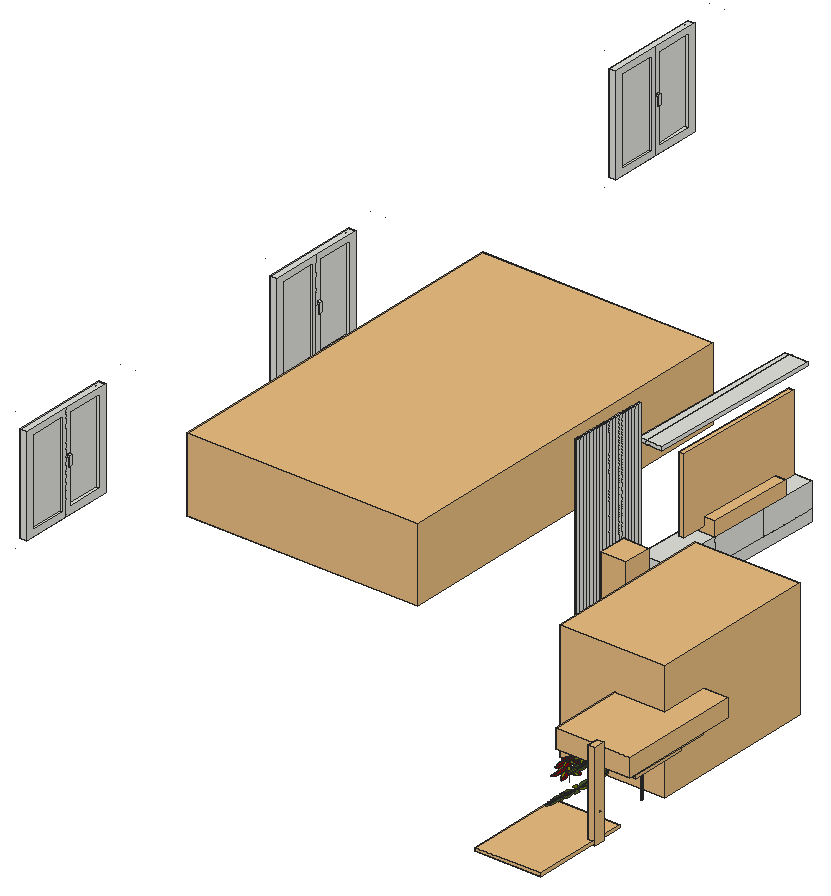
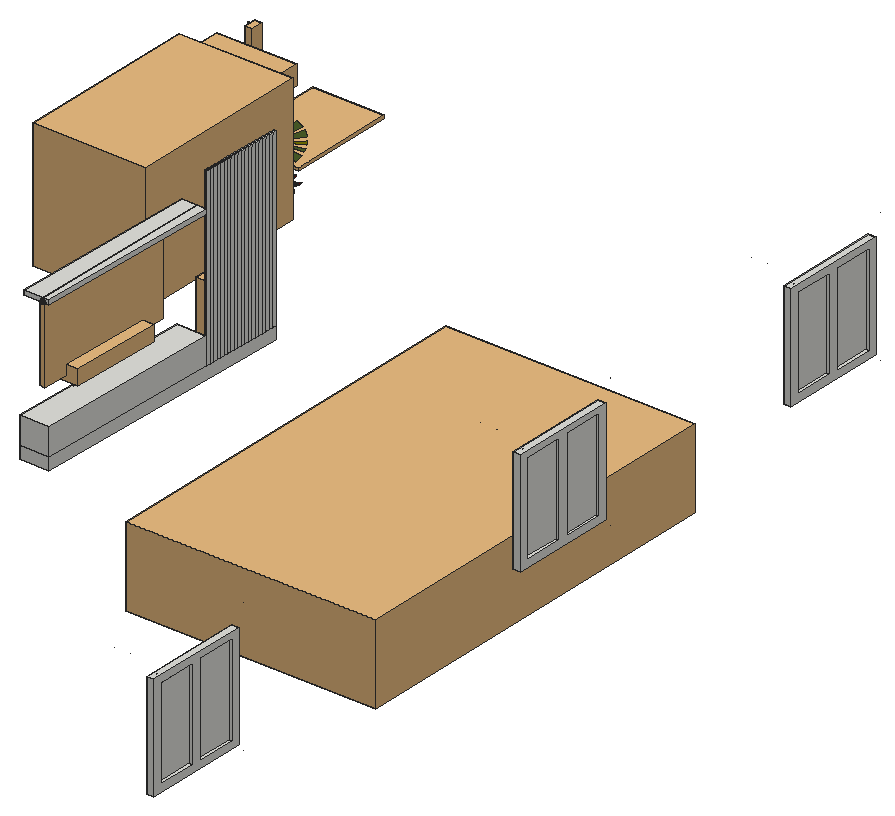
# SketchUp Ruby script. Lengths in inches.
U = 1.inch
M = Sketchup.active_model
def pt(a) = Geom::Point3d.new(a.map { |v| v * U })
def face(e, loops, mat)
  f = e.add_face(loops[0].map { |a| pt(a) })
  loops[1..].each { |l| e.add_face(l.map { |a| pt(a) }).erase! }
  f.material = f.back_material = mat if mat
  f
end
# faces: each face lists its corners as indices into pts; further lists are holes
def faces(e, pts, list, mat = nil) = list.each { |f| face(e, (f[0].is_a?(Array) ? f : [f]).map { |l| l.map { |i| pts[i] } }, mat) }
# xy, xz, yz: faces in a plane at the given z, y or x. An outline is a flat list of corners, or four numbers for a rectangle; further outlines are holes
def ring(l) = l.size == 4 ? [[l[0], l[1]], [l[2], l[1]], [l[2], l[3]], [l[0], l[3]]] : l.each_slice(2).to_a
def flat(e, list, mat, &to3) = list.each { |f| face(e, (f[0].is_a?(Array) ? f : [f]).map { |l| ring(l).map { |u, v| to3.(u, v) } }, mat) }
def xy(e, z, list, mat = nil) = flat(e, list, mat) { |x, y| [x, y, z] }
def xz(e, y, list, mat = nil) = flat(e, list, mat) { |x, z| [x, y, z] }
def yz(e, x, list, mat = nil) = flat(e, list, mat) { |y, z| [x, y, z] }
def lines(e, pts, list) = list.each { |a, b| e.add_line(pt(pts[a]), pt(pts[b])) }
# prism: a flat outline (further loops are holes) pulled along v
def prism(e, loops, v, mat = nil)
  f = face(e, loops, mat); d = Geom::Vector3d.new(v.map { |x| x * U })
  f.pushpull(f.normal.samedirection?(d) ? d.length : -d.length)
end
def box(e, o, s, mat = nil) = prism(e, [[o, [o[0] + s[0], o[1], o[2]], [o[0] + s[0], o[1] + s[1], o[2]], [o[0], o[1] + s[1], o[2]]]], [0, 0, s[2]], mat)
def at(x, y, z, deg = 0) = Geom::Transformation.translation(pt([x, y, z])) * Geom::Transformation.rotation(ORIGIN, Z_AXIS, deg.degrees)
def axes(o, x, y, z) = Geom::Transformation.new([*x, 0, *y, 0, *z, 0, *pt(o).to_a, 1])
def part(name) = M.definitions.add(name)
# library, detail: a bought-in or finely detailed component or shape, given as its bounding box
def library(name, o, s) = part(name).tap { |d| box(d.entities, o, s) }
def detail(e, o, s) = box(e.add_group.entities, o, s)
def put(e, d, t, mat = nil) = e.add_instance(d, t).tap { |i| i.material = mat if mat }
def group(e, t, mat = nil) = e.add_group.tap { |g| g.transformation = t; g.material = mat if mat }.entities
root = M.entities
M.materials.add("[0022_Maroon]").color = [128, 0, 0]
M.materials.add("[0043_SaddleBrown]").color = [139, 69, 19]
M.materials.add("[0058_Olive]").color = [128, 128, 0]
M.materials.add("[0059_DarkOliveGreen]").color = [85, 107, 47]
M.materials.add("[Metal_Aluminum_Anodized]").color = [200, 209, 218]
c1 = library("EXOTIC-AMAZON-LILY",[-1.1,-0.12,0],[60.56,66.69,1.97])
c2 = library("EXOTIC-BULLRUSH",[-0.59,-0.59,-0.94],[7.09,7.09,64.29])
c3 = part("Group\#129")
p = [[9.84,8.91,4.16],[6.8,0.43,0.2],[7.02,0.37,0.17],[7.24,0.3125,0.15],[7.46,0.26,0.12],[7.68,0.21,0.1],
  [7.91,0.17,0.08],[8.13,0.13,0.0625],[8.36,0.1,0.04],[8.59,0.07,0.03],[8.8125,0.04,0.02],[9.04,0.02,0.01],
  [9.27,0.01,0],[9.5,0,0],[10.87,0.04,0.02],[11.1,0.07,0.03],[11.33,0.1,0.04],[11.55,0.13,0.0625],
  [11.78,0.17,0.08],[12,0.21,0.1],[12.22,0.26,0.12],[12.45,0.3125,0.15],[12.67,0.37,0.17],[12.88,0.43,0.2],
  [13.1,0.5,0.23],[13.32,0.57,0.27],[13.53,0.64,0.3],[4.34,1.52,0.71],[4.43,1.46,0.68],[4.53,1.41,0.66],
  [4.625,1.35,0.63],[4.72,1.3,0.6],[4.82,1.24,0.58],[4.92,1.19,0.55],[5.02,1.14,0.53],[5.12,1.09,0.51],
  [5.22,1.04,0.48],[5.32,0.99,0.46],[5.43,0.94,0.44],[5.53,0.9,0.42],[14.76,1.19,0.55],[14.86,1.24,0.58],
  [14.96,1.3,0.6],[15.06,1.35,0.63],[15.16,1.41,0.66],[15.25,1.46,0.68],[15.35,1.52,0.71],[15.44,1.58,0.74],
  [15.53,1.64,0.76],[15.63,1.7,0.79],[15.72,1.76,0.82],[15.8125,1.82,0.85],[15.9,1.89,0.88],[1.5,4.1875,1.95],
  [1.62,4.01,1.87],[1.75,3.84,1.79],[1.88,3.67,1.71],[2.02,3.51,1.63],[2.16,3.34,1.56],[2.3,3.18,1.48],
  [2.45,3.02,1.41],[2.61,2.87,1.34],[2.76,2.72,1.27],[2.92,2.57,1.2],[3.09,2.43,1.13],[3.26,2.29,1.07],
  [17.81,3.67,1.71],[17.74,3.59,1.67],[17.67,3.51,1.63],[17.6,3.42,1.6],[17.53,3.34,1.56],[17.46,3.26,1.52],
  [17.38,3.18,1.48],[17.31,3.1,1.45],[17.23,3.02,1.41],[17.16,2.95,1.375],[17.08,2.87,1.34],[17,2.79,1.3],
  [16.92,2.72,1.27],[18.53,4.73,2.2],[18.64,4.91,2.29],[18.74,5.1,2.38],[18.83,5.29,2.47],[18.92,5.48,2.55],
  [19.01,5.67,2.64],[19.09,5.86,2.73],[19.17,6.06,2.83],[19.24,6.26,2.92],[19.3,6.46,3.01],[19.36,6.66,3.1],
  [19.42,6.86,3.2],[19.47,7.06,3.29],[0.1,7.67,3.58],[0.13,7.47,3.48],[0.17,7.26,3.39],[0.22,7.06,3.29],
  [0.27,6.86,3.2],[0.32,6.66,3.1],[0.38,6.46,3.01],[0.45,6.26,2.92],[0.52,6.06,2.83],[0.59,5.86,2.73],
  [0.67,5.67,2.64],[0.76,5.48,2.55],[0.85,5.29,2.47],[19.66,8.29,3.87],[19.67,8.5,3.96],[19.68,8.71,4.06],
  [19.69,8.91,4.16],[19.68,9.12,4.25],[19.67,9.33,4.35],[19.66,9.54,4.45],[19.64,9.74,4.54],[19.62,9.95,4.64],
  [19.59,10.16,4.74],[19.55,10.36,4.83],[19.51,10.57,4.93],[19.47,10.77,5.02],[0.1,10.16,4.74],[0.08,10.05,4.6875],
  [0.07,9.95,4.64],[0.05,9.85,4.59],[0.04,9.74,4.54],[0.03,9.64,4.5],[0.02,9.54,4.45],[0.02,9.43,4.4],
  [0.01,9.33,4.35],[0.01,9.23,4.3],[0,9.12,4.25],[0,9.02,4.21],[0,8.91,4.16],[0.85,12.54,5.85],
  [0.8,12.45,5.8],[0.76,12.35,5.76],[0.72,12.26,5.72],[0.67,12.16,5.67],[0.63,12.0625,5.625],[0.59,11.97,5.58],
  [0.56,11.87,5.53],[0.52,11.77,5.49],[0.48,11.67,5.44],[0.45,11.57,5.4],[0.41,11.47,5.35],[0.38,11.375,5.3],
  [3.26,15.54,7.25],[3.09,15.4,7.18],[2.92,15.26,7.12],[2.76,15.11,7.05],[2.61,14.96,6.98],[2.45,14.81,6.9],
  [2.3,14.65,6.83],[2.16,14.49,6.76],[2.02,14.32,6.68],[1.88,14.16,6.6],[1.75,13.99,6.52],[1.62,13.82,6.44],
  [1.5,13.64,6.36],[6.8,17.4,8.11],[6.58,17.33,8.08],[6.37,17.26,8.05],[6.16,17.1875,8.01],[5.94,17.11,7.98],
  [5.73,17.02,7.9375],[5.53,16.93,7.9],[5.32,16.84,7.85],[5.12,16.74,7.81],[4.92,16.64,7.76],[4.72,16.53,7.71],
  [4.53,16.42,7.66],[4.34,16.31,7.61],[9.5,17.83,8.3125],[9.38,17.83,8.3125],[9.27,17.82,8.31],[9.16,17.8125,8.31],
  [9.04,17.81,8.3],[8.93,17.8,8.3],[8.8125,17.79,8.29],[8.7,17.77,8.29],[8.59,17.76,8.28],[8.47,17.75,8.28],
  [8.36,17.73,8.27],[8.25,17.72,8.26],[8.13,17.7,8.25],[19.09,11.97,5.58],[19.05,12.0625,5.625],[19.01,12.16,5.67],
  [18.97,12.26,5.72],[18.92,12.35,5.76],[18.88,12.45,5.8],[18.83,12.54,5.85],[18.79,12.64,5.89],[18.74,12.73,5.9375],
  [18.6875,12.83,5.98],[18.64,12.92,6.02],[18.59,13.01,6.07],[18.53,13.1,6.11],[16.92,15.11,7.05],[17,15.04,7.01],
  [17.08,14.96,6.98],[17.16,14.88,6.94],[17.23,14.81,6.9],[17.31,14.73,6.87],[17.38,14.65,6.83],[17.46,14.57,6.79],
  [17.53,14.49,6.76],[17.6,14.41,6.72],[17.67,14.32,6.68],[17.74,14.24,6.64],[17.81,14.16,6.6],[15.9,15.94,7.43],
  [15.8125,16.01,7.46],[15.72,16.07,7.49],[15.63,16.13,7.52],[15.53,16.19,7.55],[15.44,16.25,7.58],[15.35,16.31,7.61],
  [15.25,16.37,7.63],[15.16,16.42,7.66],[15.06,16.48,7.68],[14.96,16.53,7.71],[14.86,16.59,7.73],[14.76,16.64,7.76],
  [13.53,17.1875,8.01],[13.32,17.26,8.05],[13.1,17.33,8.08],[12.88,17.4,8.11],[12.67,17.46,8.14],[12.45,17.52,8.17],
  [12.22,17.57,8.19],[12,17.62,8.22],[11.78,17.66,8.24],[11.55,17.7,8.25],[11.33,17.73,8.27],[11.1,17.76,8.28],
  [10.87,17.79,8.29]]
faces(c3.entities,p,[[0,1,2,3,4,5,6,7,8,9,10,11,12,13],[0,14,15,16,17,18,19,20,21,22,23,24,25,26],[0,40,41,42,43,44,45,46,47,48,49,50,51,52],[0,53,54,55,56,57,58,59,60,61,62,63,64,65],[0,79,80,81,82,83,84,85,86,87,88,89,90,91],[0,92,93,94,95,96,97,98,99,100,101,102,103,104],[0,105,106,107,108,109,110,111,112,113,114,115,116,117],[0,118,119,120,121,122,123,124,125,126,127,128,129,130],
  [0,144,145,146,147,148,149,150,151,152,153,154,155,156],[0,170,171,172,173,174,175,176,177,178,179,180,181,182],[0,196,197,198,199,200,201,202,203,204,205,206,207,208],[0,209,210,211,212,213,214,215,216,217,218,219,220,221]],"[0059_DarkOliveGreen]")
faces(c3.entities,p,[[0,27,28,29,30,31,32,33,34,35,36,37,38,39],[0,66,67,68,69,70,71,72,73,74,75,76,77,78],[0,131,132,133,134,135,136,137,138,139,140,141,142,143],[0,157,158,159,160,161,162,163,164,165,166,167,168,169],[0,183,184,185,186,187,188,189,190,191,192,193,194,195],[0,222,223,224,225,226,227,228,229,230,231,232,233,234]],"[0058_Olive]")
c4 = part("EXOTIC-AUS-PALM")
put(c4.entities,c3,axes([-13.78,-12.48,-5.82],[1.4,0,0],[0,1.4,0],[0,0,1.4]))
put(c4.entities,c3,at(-21.65,-8.91,-12.03))
put(c4.entities,c3,axes([-1.28,-11.86,-13.4],[1.33,0,0],[0,1.33,0],[0,0,1.33]))
c5 = part("Group\#125")
p = [[0.46,5.4,1.48],[0.55,4.86,1.35],[0.68,4.33,1.23],[0.85,3.8,1.12],[1.04,3.28,1.02],[1.28,2.78,0.93],
  [1.54,2.29,0.84],[1.84,1.82,0.77],[2.17,1.36,0.71],[2.52,0.93,0.66],[2.91,0.52,0.62],[2.91,0,0.48],
  [2.47,0.44,0.52],[2.06,0.9,0.56],[1.68,1.39,0.625],[1.34,1.9,0.7],[1.03,2.43,0.79],[0.76,2.98,0.89],
  [0.53,3.55,1],[0.34,4.13,1.12],[0.19,4.72,1.25],[0.09,5.3125,1.39],[0.02,5.91,1.54],[0,6.51,1.69],
  [0.02,6.88,1.8],[0.1,7.24,1.91],[0.22,7.59,2.02],[0.39,7.92,2.14],[0.6,8.22,2.26],[0.85,8.49,2.38],
  [1.14,8.72,2.49],[1.45,8.91,2.6],[1.8,9.0625,2.71],[2.16,9.17,2.8],[2.53,9.22,2.88],[2.91,9.23,2.95],
  [2.91,4.61,1.72],[2.68,3.89,1.48],[2.18,2.26,0.95],[2.59,5.625,1.93],[1.61,4.02,1.32],[2.34,6.73,2.18],
  [1.25,5.66,1.69],[2.4,7.87,2.5],[1.14,7.72,2.22],[2.4375,8.83,2.76],[2.16,8.77,2.69],[1.89,8.68,2.62],
  [1.625,8.56,2.54],[1.39,8.42,2.46],[1.16,8.24,2.37],[0.97,8.04,2.28],[0.79,7.82,2.19],[0.65,7.58,2.1],
  [0.54,7.32,2.01],[0.45,7.05,1.92],[0.4,6.78,1.84],[0.39,6.49,1.76],[0.41,5.95,1.62],[5.79,6.88,1.8],
  [5.82,6.51,1.69],[5.79,5.91,1.54],[5.73,5.3125,1.39],[5.625,4.72,1.25],[5.48,4.13,1.12],[5.29,3.55,1],
  [5.06,2.98,0.89],[4.79,2.43,0.79],[4.48,1.9,0.7],[4.14,1.39,0.625],[3.76,0.9,0.56],[3.35,0.44,0.52],
  [3.29,0.93,0.66],[3.65,1.36,0.71],[3.98,1.82,0.77],[4.27,2.29,0.84],[4.54,2.78,0.93],[4.77,3.28,1.02],
  [4.97,3.8,1.12],[5.13,4.33,1.23],[5.26,4.86,1.35],[5.35,5.4,1.48],[5.41,5.95,1.62],[5.43,6.49,1.76],
  [5.41,6.78,1.84],[5.36,7.05,1.92],[5.28,7.32,2.01],[5.16,7.58,2.1],[5.02,7.82,2.19],[4.85,8.04,2.28],
  [4.65,8.24,2.37],[4.43,8.42,2.46],[4.1875,8.56,2.54],[3.93,8.68,2.62],[3.66,8.77,2.69],[3.38,8.83,2.76],
  [4.67,7.72,2.22],[3.41,7.87,2.5],[4.5625,5.66,1.69],[3.47,6.73,2.18],[4.21,4.02,1.32],[3.23,5.625,1.93],
  [3.64,2.26,0.95],[3.13,3.89,1.48],[3.29,9.22,2.88],[3.66,9.17,2.8],[4.02,9.0625,2.71],[4.36,8.91,2.6],
  [4.68,8.72,2.49],[4.96,8.49,2.38],[5.21,8.22,2.26],[5.43,7.92,2.14],[5.59,7.59,2.02],[5.72,7.24,1.91],
  [2.91,14.34,0]]
faces(c5.entities,p,[[0,1,2,3,4,5,6,7,8,9,10,11,12,13,14,15,16,17,18,19,20,21,22,23,24,25,26,27,28,29,30,31,32,33,34,35,36,10,37,38,39,40,41,42,43,44,45,46,47,48,49,50,51,52,53,54,55,56,57,58],[59,60,61,62,63,64,65,66,67,68,69,70,71,11,10,72,73,74,75,76,77,78,79,80,81,82,83,84,85,86,87,88,89,90,91,92,93,94,95,96,97,98,99,100,101,102,103,10,36,35,104,105,106,107,108,109,110,111,112,113]],"[0022_Maroon]")
faces(c5.entities,p,[[43,42,41,40,39,38,37,10,9,8,7,6,5,4,3,2,1,0,58,57,56,55,54,53,52,51,50,49,48,47,46,45,44],[99,98,97,96,95,94,93,92,91,90,89,88,87,86,85,84,83,82,81,80,79,78,77,76,75,74,73,72,10,103,102,101,100]],"[0058_Olive]")
lines(c5.entities,p,[[35,114]])
c6 = part("EXOTIC-CROTON")
p = [[0,0,13.11],[0,0,0],[0,0,17.6]]
lines(c6.entities,p,[[0,1],[0,2]])
put(c6.entities,c5,at(-2.91,-14.34,9.43),"[0058_Olive]")
put(c6.entities,c5,at(-13.875,-4.65,9.43,-60),"[0058_Olive]")
put(c6.entities,c5,at(-10.97,9.69,9.43,-120),"[0058_Olive]")
put(c6.entities,c5,at(2.91,14.34,9.43,180),"[0058_Olive]")
put(c6.entities,c5,at(13.875,4.65,9.43,120),"[0058_Olive]")
put(c6.entities,c5,at(10.97,-9.69,9.43,60),"[0058_Olive]")
put(c6.entities,c5,axes([-3.96,11.79,13.11],[-0.73612,-0.425,0],[0.425,-0.73612,0],[0,0,0.85]),"[0058_Olive]")
put(c6.entities,c5,axes([8.24,9.32,13.11],[-0.73612,0.425,0],[-0.425,-0.73612,0],[0,0,0.85]),"[0058_Olive]")
put(c6.entities,c5,axes([3.96,-11.79,13.11],[0.73612,0.425,0],[-0.425,0.73612,0],[0,0,0.85]),"[0058_Olive]")
put(c6.entities,c5,axes([-8.24,-9.32,13.11],[0.73612,-0.425,0],[0.425,0.73612,0],[0,0,0.85]),"[0058_Olive]")
put(c6.entities,c5,axes([12.19,-2.47,13.11],[0,0.85,0],[-0.85,0,0],[0,0,0.85]),"[0058_Olive]")
put(c6.entities,c5,axes([-12.19,2.47,13.11],[0,-0.85,0],[0.85,0,0],[0,0,0.85]),"[0058_Olive]")
put(c6.entities,c5,axes([1.98,9.75,17.6],[-0.68,0,0],[0,-0.68,0],[0,0,0.68]),"[0058_Olive]")
put(c6.entities,c5,axes([7.46,-6.59,17.6],[0.34,0.5889,0],[-0.5889,0.34,0],[0,0,0.68]),"[0058_Olive]")
put(c6.entities,c5,axes([9.4375,3.16,17.6],[-0.34,0.5889,0],[-0.5889,-0.34,0],[0,0,0.68]),"[0058_Olive]")
put(c6.entities,c5,axes([-9.4375,-3.16,17.6],[0.34,-0.5889,0],[0.5889,0.34,0],[0,0,0.68]),"[0058_Olive]")
put(c6.entities,c5,axes([-7.46,6.59,17.6],[-0.34,-0.5889,0],[0.5889,-0.34,0],[0,0,0.68]),"[0058_Olive]")
put(c6.entities,c5,axes([-1.98,-9.75,17.6],[0.68,0,0],[0,0.68,0],[0,0,0.68]),"[0058_Olive]")
c7 = part("Group\#126")
p = [[12.14,1.93,0.52],[12.15,1.96,0.53]]
lines(c7.entities,p,[[0,1]])
detail(c7.entities,[0,0,0],[22.29,22.29,3.9])
c8 = part("EXOTIC-BUSHY-02")
prism(c8.entities,[[[-0.2,0.11,-0.03],[-0.16,0.16,-0.03],[-0.11,0.2,-0.03],[-0.06,0.22,-0.03],[0,0.23,-0.03],[0.06,0.22,-0.03],[0.11,0.2,-0.03],[0.16,0.16,-0.03],[0.2,0.11,-0.03],[0.22,0.06,-0.03],[0.23,0,-0.03],[0.22,-0.06,-0.03],[0.2,-0.11,-0.03],[0.16,-0.16,-0.03],[0.11,-0.2,-0.03],[0.06,-0.22,-0.03],[0,-0.23,-0.03],[-0.06,-0.22,-0.03],[-0.11,-0.2,-0.03],[-0.16,-0.16,-0.03],[-0.2,-0.11,-0.03],[-0.22,-0.06,-0.03],[-0.23,0,-0.03],[-0.22,0.06,-0.03]]],[0,0,12.79],"[0043_SaddleBrown]")
put(c8.entities,c7,axes([-11.15,-11.15,16.66],[1,0,0],[0,1,0],[0,0,-1]))
put(c8.entities,c7,axes([-7.91,-7.91,13.14],[0.71,0,0],[0,0.71,0],[0,0,-0.71]))
put(c8.entities,c7,axes([-5.11,-5.11,9.7],[0.4588,0,0],[0,0.4588,0],[0,0,-0.4588]))
c9 = part("Window")
xy(c9.entities,31.72,[[-0.78,88.6,2.72,128.1]])
xy(c9.entities,34.95,[[-0.78,91.53,0.84,106.59],[0.84,91.53,1.05,97.58],[1.05,91.53,1.42,106.59],[1.42,91.53,2.72,106.59],[0.84,97.58,1.05,98.18],
  [0.84,98.18,1.05,106.59]])
xy(c9.entities,35.27,[[-0.78,110.09,0.97,125.14],[1.05,110.09,2.72,125.14]])
xy(c9.entities,58.35,[[2.72,108.74,3.8,109.74]])
xy(c9.entities,77.8125,[[-0.78,110.09,2.72,125.14],[0.97,110.09,1.05,125.14]])
xy(c9.entities,77.93,[[-0.78,91.53,0.84,106.59],[1.05,91.53,1.42,106.59],[1.42,91.53,2.72,106.59]])
xy(c9.entities,80.72,[[-0.78,88.6,2.72,128.1]])
xz(c9.entities,88.6,[[-0.78,31.72,2.72,80.72]])
xz(c9.entities,91.53,[[-0.78,34.95,0.84,77.93],[1.05,34.95,1.42,77.93],[1.42,34.95,2.72,77.93]])
xz(c9.entities,106.59,[[-0.78,34.95,0.84,77.93],[0.84,34.95,1.05,77.93],[0.84,34.95,2.72,77.93]])
xz(c9.entities,108.74,[[3.8,54.35,4.22,54.6,4.22,59.47,2.72,59.97,2.72,58.35,3.8,58.35]])
xz(c9.entities,109.74,[[3.8,54.35,3.8,58.35,2.72,58.35,2.72,59.97,4.22,59.47,4.22,54.6]])
xz(c9.entities,110.09,[[-0.78,35.27,0.97,77.8125],[1.05,35.27,2.72,77.8125]])
xz(c9.entities,125.14,[[-0.78,35.27,0.97,77.8125],[0.97,35.27,1.05,80.72],[1.05,35.27,2.72,77.8125]])
xz(c9.entities,128.1,[[-0.78,31.72,2.72,80.72]])
yz(c9.entities,-0.78,[[[88.6,31.72,128.1,80.72],[91.53,34.95,106.59,77.93],[110.09,35.27,125.14,77.8125]]])
yz(c9.entities,0.84,[[91.53,34.95,106.59,77.93]])
yz(c9.entities,0.97,[[110.09,35.27,125.14,77.8125]])
yz(c9.entities,1.05,[[91.53,34.95,106.59,77.93],[110.09,35.27,125.14,77.8125]])
yz(c9.entities,1.42,[[91.53,34.95,106.59,77.93]])
yz(c9.entities,2.72,[[[88.6,31.72,108.35,80.72],[91.53,34.95,106.59,77.93]],[[108.35,31.72,128.1,80.72],[110.09,35.27,125.14,77.8125],[108.74,58.35,109.74,59.97]]])
yz(c9.entities,3.8,[[108.74,54.35,109.74,58.35]])
yz(c9.entities,4.22,[[108.74,54.6,109.74,59.47]])
p = [[4.22,108.74,54.6],[3.8,108.74,54.35],[3.8,109.74,54.35],[4.22,109.74,54.6],[2.72,109.74,59.97],[2.72,108.74,59.97],
  [4.22,108.74,59.47],[4.22,109.74,59.47],[-0.78,86.4,89.94],[-0.78,86.44,89.94],[15.22,130.69,89.94],[15.22,130.65,89.94],
  [-0.78,86.44,28.19],[-0.78,86.4,28.19],[7.72,130.69,89.94],[7.72,130.65,89.94]]
faces(c9.entities,p,[[0,1,2,3],[4,5,6,7]])
lines(c9.entities,p,[[8,9],[10,11],[12,13],[14,15]])
c10 = library("EXOTIC-KENTIA\#1",[0.7,-0.7,-0.11],[104.19,106.14,86.09])
c11 = part("Agrupar\#1")
detail(c11.entities,[0,0,0],[43.31,13.99,7.25])
c12 = library("Agrupar\#2",[0,0,0],[66.49,2.6,38.28])
c13 = part("Samsung 75")
p = [[0,0,0],[1,0,0],[1,1,0]]
lines(c13.entities,p,[[0,1],[1,2],[2,0]])
put(c13.entities,c11,at(200.625,110.82,-2.44),"[Metal_Aluminum_Anodized]")
put(c13.entities,c12,at(189.03,116.54,0))
c14 = library("Vtufgjkbc",[-37.34,-38.3,0],[76.68,71.13,141.17])
c15 = part("Enscape.LinearLight")
xz(c15.entities,-44.64,[[0,-1,0,0,-0.38,-0.92],[0,-1,0.38,-0.92,0,0],[-0.38,-0.92,0,0,-0.71,-0.71],[0.38,-0.92,0.71,-0.71,0,0],[-0.71,-0.71,0,0,-0.92,-0.38],
  [0.71,-0.71,0.92,-0.38,0,0],[-0.92,-0.38,0,0,-1,0],[0.92,-0.38,1,0,0,0],[-1,0,0,0,-0.92,0.38],[0,0,-0.71,0.71,-0.92,0.38],
  [0,0,-0.38,0.92,-0.71,0.71],[0,0,0,1,-0.38,0.92],[0,0,0.38,0.92,0,1],[0,0,0.71,0.71,0.38,0.92],[0,0,0.92,0.38,0.71,0.71],
  [0,0,1,0,0.92,0.38]])
xz(c15.entities,44.64,[[0,-1,-0.38,-0.92,0,0],[0,-1,0,0,0.38,-0.92],[-0.38,-0.92,-0.71,-0.71,0,0],[0.38,-0.92,0,0,0.71,-0.71],[-0.71,-0.71,-0.92,-0.38,0,0],
  [0.71,-0.71,0,0,0.92,-0.38],[-0.92,-0.38,-1,0,0,0],[0.92,-0.38,0,0,1,0],[-1,0,-0.92,0.38,0,0],[0,0,-0.92,0.38,-0.71,0.71],
  [0,0,-0.71,0.71,-0.38,0.92],[0,0,-0.38,0.92,0,1],[0,0,0,1,0.38,0.92],[0,0,0.38,0.92,0.71,0.71],[0,0,0.71,0.71,0.92,0.38],
  [0,0,0.92,0.38,1,0]])
p = [[-0.38,-44.64,-0.92],[-0.38,44.64,-0.92],[0,44.64,-1],[0,-44.64,-1],[0.38,44.64,-0.92],[0.38,-44.64,-0.92],
  [-0.71,-44.64,-0.71],[-0.71,44.64,-0.71],[0.71,44.64,-0.71],[0.71,-44.64,-0.71],[-0.92,-44.64,-0.38],[-0.92,44.64,-0.38],
  [0.92,44.64,-0.38],[0.92,-44.64,-0.38],[-1,-44.64,0],[-1,44.64,0],[1,44.64,0],[1,-44.64,0],
  [-0.92,-44.64,0.38],[-0.92,44.64,0.38],[0.92,44.64,0.38],[0.92,-44.64,0.38],[-0.71,-44.64,0.71],[-0.71,44.64,0.71],
  [0.71,44.64,0.71],[0.71,-44.64,0.71],[-0.38,-44.64,0.92],[-0.38,44.64,0.92],[0.38,44.64,0.92],[0.38,-44.64,0.92],
  [0,-44.64,1],[0,44.64,1]]
faces(c15.entities,p,[[0,1,2],[0,2,3],[3,2,4],[3,4,5],[6,7,1],[6,1,0],[5,4,8],[5,8,9],
  [10,11,7],[10,7,6],[9,8,12],[9,12,13],[14,15,11],[14,11,10],[13,12,16],[13,16,17],
  [18,19,15],[18,15,14],[17,16,20],[17,20,21],[22,23,19],[22,19,18],[21,20,24],[21,24,25],
  [26,27,23],[26,23,22],[25,24,28],[25,28,29],[30,31,27],[30,27,26],[29,28,31],[29,31,30]])
c16 = part("Group\#8")
box(c16.entities,[0,0,0],[1.57,1.18,81.22])
c17 = part("tv unit")
put(c17.entities,c13,at(-134.98,-45.95,38.54))
put(c17.entities,c14,axes([23.51,76.07,18.38],[0.185,0,0],[0,0.185,0],[0,0,0.185]))
put(c17.entities,c15,axes([87.75,81.2,82.67],[-0.0192,0.99911,-0.03748],[-0.99982,-0.01919,0.00072],[0,0.03749,0.9993]))
g1 = group(c17.entities,at(3.9375,84.65,12.68))
box(g1,[0,-13.78,0],[127.95,13.78,5.79])
g2 = group(c17.entities,at(43.31,84.65,18.46))
prism(g2,[[[0,0,0],[88.58,0,0],[88.58,-13.78,0],[59.21,-13.78,0],[59.21,-12.99,0],[59.06,-12.99,0],[59.06,-13.78,0],[29.69,-13.78,0],[29.69,-12.99,0],[29.53,-12.99,0],[29.53,-13.78,0],[0,-13.78,0]]],[0,0,12.6])
g3 = group(c17.entities,at(3.9375,84.65,18.46))
put(g3,c16,at(0,-1.18,0))
g4 = group(g3,at(1.97,-1.18,0))
box(g4,[0,0,0],[1.57,1.18,81.22])
put(g3,c16,at(3.9375,-1.18,0))
put(g3,c16,at(5.91,-1.18,0))
g5 = group(g3,at(7.875,-1.18,0))
box(g5,[0,0,0],[1.57,1.18,81.22])
put(g3,c16,at(9.84,-1.18,0))
put(g3,c16,at(11.8125,-1.18,0))
put(g3,c16,at(13.78,-1.18,0))
put(g3,c16,at(15.75,-1.18,0))
put(g3,c16,at(17.72,-1.18,0))
put(g3,c16,at(19.69,-1.18,0))
put(g3,c16,at(21.65,-1.18,0))
put(g3,c16,at(23.62,-1.18,0))
g6 = group(g3,at(25.59,-1.18,0))
box(g6,[0,0,0],[1.57,1.18,81.22])
put(g3,c16,at(27.56,-1.18,0))
put(g3,c16,at(29.53,-1.18,0))
put(g3,c16,at(31.5,-1.18,0))
put(g3,c16,at(33.46,-1.18,0))
put(g3,c16,at(35.43,-1.18,0))
put(g3,c16,at(37.4,-1.18,0))
g7 = group(c17.entities,at(42.91,84.65,81.97))
box(g7,[0,-11.8125,0],[88.98,11.8125,1.97])
c18 = library("Sofa\#1",[-63.29,58.08,-3.15],[123.29,84.21,37.08])
put(root,c1,axes([272.96,125.26,9.51],[0,-0.82,0],[0.49713,0,0],[0,0,0.69]))
put(root,c2,axes([303.48,114.89,9.51],[0,-0.82,0],[0.49713,0,0],[0,0,0.69]))
put(root,c4,axes([283.18,142.31,26.63],[0,-1.23,0],[0.74569,0,0],[0,0,1.035]))
put(root,c6,axes([265.35,145.17,7.39],[0,-0.64206,0],[0.38925,0,0],[0,0,0.54027]))
put(root,c8,axes([298.27,149.71,9.55],[0,-2.7716,0],[1.68028,0,0],[0,0,2.3322]))
put(root,c9,axes([0.78,20.35,-0.95],[1,0,0],[0,1.25,0],[0,0,1]))
put(root,c6,axes([266.9,156.5625,9.51],[0,-0.82,0],[0.49713,0,0],[0,0,0.69]))
put(root,c6,axes([265.35,167.74,7.39],[0,-0.64206,0],[0.38925,0,0],[0,0,0.54027]))
put(root,c10,axes([252.08,242.17,9.51],[0,-0.82,0],[0.49713,0,0],[0,0,0.69]))
put(root,c17,at(281.93,227.23,0,88.4))
put(root,c9,axes([0.78,177.79,-0.95],[1,0,0],[0,1.25,0],[0,0,1]))
put(root,c18,axes([-71.15,315.52,5.99],[0,-1.50871,0],[1.38,0,0],[0,0,1]))
put(root,c9,axes([0.78,391.23,-0.95],[1,0,0],[0,1.25,0],[0,0,1]))
